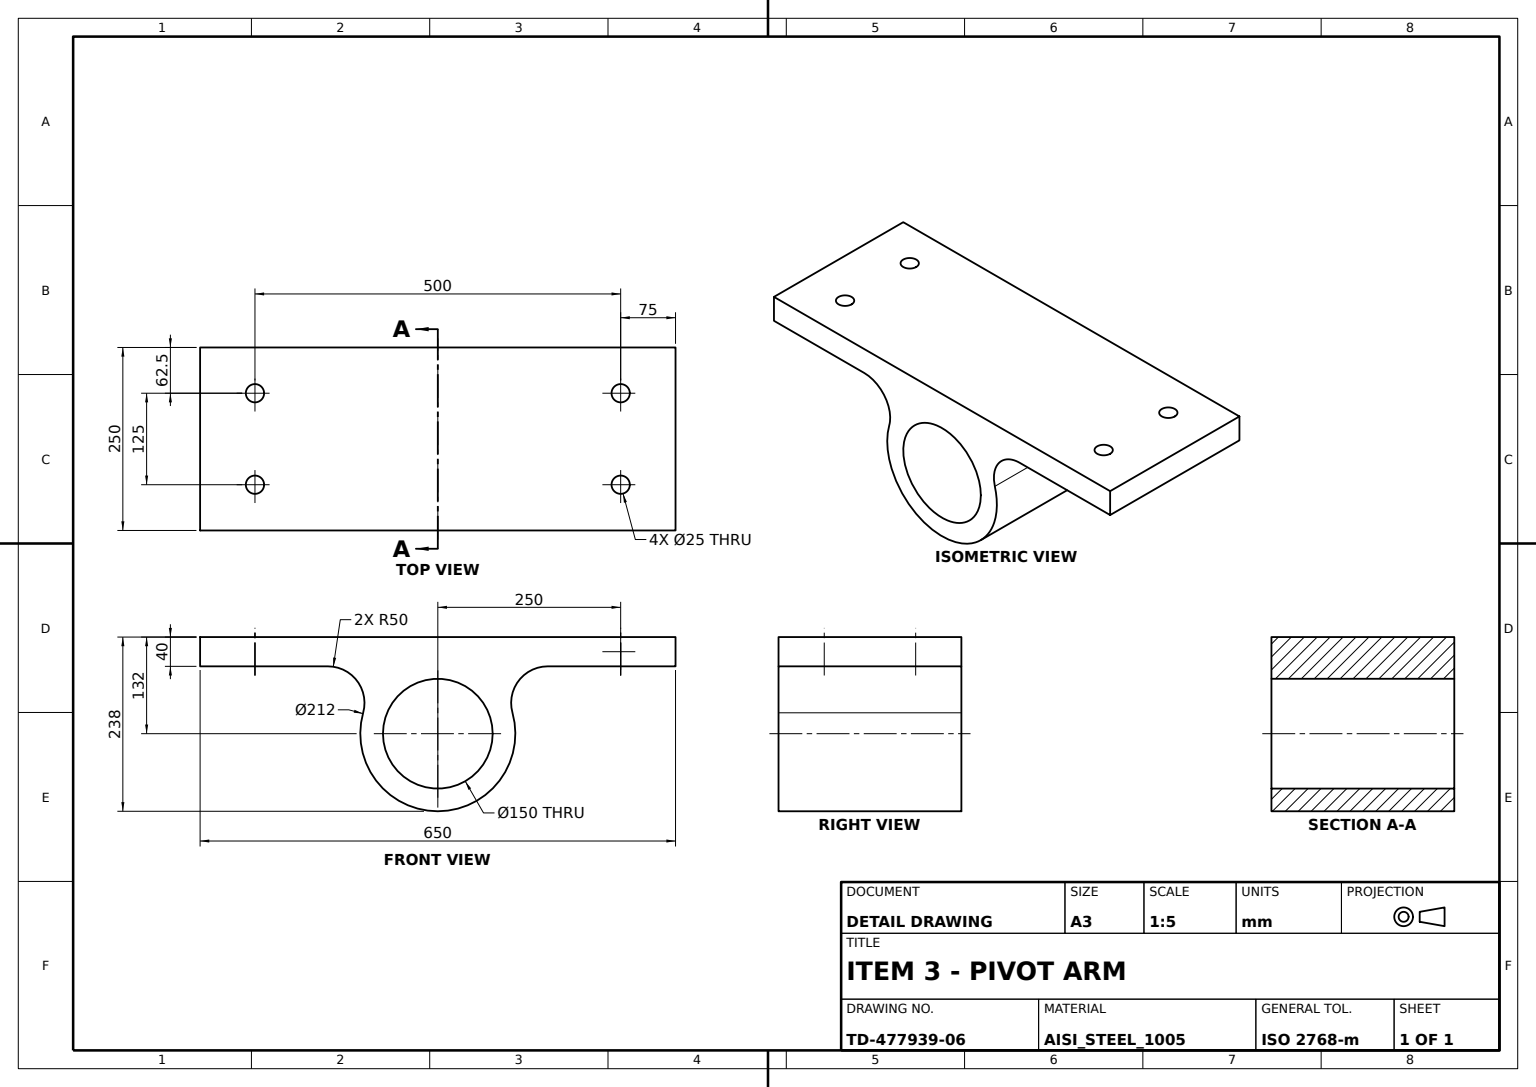
ISO-10303-21;
HEADER;
FILE_DESCRIPTION((''),'2;1');
FILE_NAME('','',(''),(''),'','','');
FILE_SCHEMA(('AUTOMOTIVE_DESIGN'));
ENDSEC;
DATA;
#1=APPLICATION_CONTEXT('');
#2=PRODUCT_CONTEXT('',#1,'mechanical');
#3=PRODUCT('','','',(#2));
#4=PRODUCT_DEFINITION_FORMATION('','',#3);
#5=PRODUCT_DEFINITION_CONTEXT('',#1,'design');
#6=PRODUCT_DEFINITION('','',#4,#5);
#7=PRODUCT_DEFINITION_SHAPE('','',#6);
#8=(LENGTH_UNIT()NAMED_UNIT(*)SI_UNIT(.MILLI.,.METRE.));
#9=(NAMED_UNIT(*)PLANE_ANGLE_UNIT()SI_UNIT($,.RADIAN.));
#10=(NAMED_UNIT(*)SI_UNIT($,.STERADIAN.)SOLID_ANGLE_UNIT());
#11=UNCERTAINTY_MEASURE_WITH_UNIT(LENGTH_MEASURE(0.005),#8,'distance_accuracy_value','');
#12=(GEOMETRIC_REPRESENTATION_CONTEXT(3)GLOBAL_UNCERTAINTY_ASSIGNED_CONTEXT((#11))GLOBAL_UNIT_ASSIGNED_CONTEXT((#8,#9,#10))REPRESENTATION_CONTEXT('',''));
#13=CARTESIAN_POINT('',(125.,-102.086024,28.538462));
#14=VERTEX_POINT('',#13);
#15=CARTESIAN_POINT('',(125.,102.086024,28.538462));
#16=VERTEX_POINT('',#15);
#17=CARTESIAN_POINT('',(125.,0.,0.));
#18=DIRECTION('',(1.,0.,0.));
#19=DIRECTION('',(0.,1.,0.));
#20=AXIS2_PLACEMENT_3D('',#17,#18,#19);
#21=CIRCLE('',#20,106.);
#22=EDGE_CURVE('',#14,#16,#21,.T.);
#23=ORIENTED_EDGE('',*,*,#22,.F.);
#24=CARTESIAN_POINT('',(-125.,-102.086024,28.538462));
#25=VERTEX_POINT('',#24);
#26=DIRECTION('',(-1.,0.,0.));
#27=VECTOR('',#26,1000.);
#28=LINE('',#13,#27);
#29=EDGE_CURVE('',#14,#25,#28,.T.);
#30=ORIENTED_EDGE('',*,*,#29,.T.);
#31=CARTESIAN_POINT('',(-125.,102.086024,28.538462));
#32=VERTEX_POINT('',#31);
#33=CARTESIAN_POINT('',(-125.,0.,0.));
#34=AXIS2_PLACEMENT_3D('',#33,#18,#19);
#35=CIRCLE('',#34,106.);
#36=EDGE_CURVE('',#25,#32,#35,.T.);
#37=ORIENTED_EDGE('',*,*,#36,.T.);
#38=LINE('',#15,#27);
#39=EDGE_CURVE('',#16,#32,#38,.T.);
#40=ORIENTED_EDGE('',*,*,#39,.F.);
#41=EDGE_LOOP('',(#23,#30,#37,#40));
#42=FACE_BOUND('',#41,.T.);
#43=DIRECTION('',(0.,0.,1.));
#44=AXIS2_PLACEMENT_3D('',#17,#26,#43);
#45=CYLINDRICAL_SURFACE('',#44,106.);
#46=ADVANCED_FACE('',(#42),#45,.T.);
#47=CARTESIAN_POINT('',(-125.,325.,132.));
#48=VERTEX_POINT('',#47);
#49=CARTESIAN_POINT('',(-125.,-325.,132.));
#50=VERTEX_POINT('',#49);
#51=DIRECTION('',(0.,-1.,0.));
#52=VECTOR('',#51,1000.);
#53=LINE('',#47,#52);
#54=EDGE_CURVE('',#48,#50,#53,.T.);
#55=ORIENTED_EDGE('',*,*,#54,.T.);
#56=CARTESIAN_POINT('',(125.,-325.,132.));
#57=VERTEX_POINT('',#56);
#58=LINE('',#56,#27);
#59=EDGE_CURVE('',#57,#50,#58,.T.);
#60=ORIENTED_EDGE('',*,*,#59,.F.);
#61=CARTESIAN_POINT('',(125.,325.,132.));
#62=VERTEX_POINT('',#61);
#63=LINE('',#61,#52);
#64=EDGE_CURVE('',#62,#57,#63,.T.);
#65=ORIENTED_EDGE('',*,*,#64,.F.);
#66=LINE('',#61,#27);
#67=EDGE_CURVE('',#62,#48,#66,.T.);
#68=ORIENTED_EDGE('',*,*,#67,.T.);
#69=EDGE_LOOP('',(#55,#60,#65,#68));
#70=FACE_BOUND('',#69,.T.);
#71=CARTESIAN_POINT('',(-62.5,-237.5,132.));
#72=VERTEX_POINT('',#71);
#73=CARTESIAN_POINT('',(-62.5,-250.,132.));
#74=AXIS2_PLACEMENT_3D('',#73,#43,#19);
#75=CIRCLE('',#74,12.5);
#76=EDGE_CURVE('',#72,#72,#75,.T.);
#77=ORIENTED_EDGE('',*,*,#76,.F.);
#78=EDGE_LOOP('',(#77));
#79=FACE_BOUND('',#78,.T.);
#80=CARTESIAN_POINT('',(62.5,-237.5,132.));
#81=VERTEX_POINT('',#80);
#82=CARTESIAN_POINT('',(62.5,-250.,132.));
#83=AXIS2_PLACEMENT_3D('',#82,#43,#19);
#84=CIRCLE('',#83,12.5);
#85=EDGE_CURVE('',#81,#81,#84,.T.);
#86=ORIENTED_EDGE('',*,*,#85,.F.);
#87=EDGE_LOOP('',(#86));
#88=FACE_BOUND('',#87,.T.);
#89=CARTESIAN_POINT('',(-62.5,262.5,132.));
#90=VERTEX_POINT('',#89);
#91=CARTESIAN_POINT('',(-62.5,250.,132.));
#92=AXIS2_PLACEMENT_3D('',#91,#43,#19);
#93=CIRCLE('',#92,12.5);
#94=EDGE_CURVE('',#90,#90,#93,.T.);
#95=ORIENTED_EDGE('',*,*,#94,.F.);
#96=EDGE_LOOP('',(#95));
#97=FACE_BOUND('',#96,.T.);
#98=CARTESIAN_POINT('',(62.5,262.5,132.));
#99=VERTEX_POINT('',#98);
#100=CARTESIAN_POINT('',(62.5,250.,132.));
#101=AXIS2_PLACEMENT_3D('',#100,#43,#19);
#102=CIRCLE('',#101,12.5);
#103=EDGE_CURVE('',#99,#99,#102,.T.);
#104=ORIENTED_EDGE('',*,*,#103,.F.);
#105=EDGE_LOOP('',(#104));
#106=FACE_BOUND('',#105,.T.);
#107=DIRECTION('',(0.,0.,-1.));
#108=AXIS2_PLACEMENT_3D('',#61,#107,#26);
#109=PLANE('',#108);
#110=ADVANCED_FACE('',(#70,#79,#88,#97,#106),#109,.F.);
#111=ORIENTED_EDGE('',*,*,#103,.T.);
#112=EDGE_LOOP('',(#111));
#113=FACE_BOUND('',#112,.T.);
#114=CARTESIAN_POINT('',(75.,250.,92.));
#115=VERTEX_POINT('',#114);
#116=CARTESIAN_POINT('',(62.5,250.,92.));
#117=AXIS2_PLACEMENT_3D('',#116,#43,#18);
#118=CIRCLE('',#117,12.5);
#119=EDGE_CURVE('',#115,#115,#118,.T.);
#120=ORIENTED_EDGE('',*,*,#119,.F.);
#121=EDGE_LOOP('',(#120));
#122=FACE_BOUND('',#121,.T.);
#123=CARTESIAN_POINT('',(62.5,250.,7.));
#124=AXIS2_PLACEMENT_3D('',#123,#43,#18);
#125=CYLINDRICAL_SURFACE('',#124,12.5);
#126=ADVANCED_FACE('',(#113,#122),#125,.F.);
#127=ORIENTED_EDGE('',*,*,#119,.T.);
#128=EDGE_LOOP('',(#127));
#129=FACE_BOUND('',#128,.T.);
#130=CARTESIAN_POINT('',(-50.,250.,92.));
#131=VERTEX_POINT('',#130);
#132=CARTESIAN_POINT('',(-62.5,250.,92.));
#133=AXIS2_PLACEMENT_3D('',#132,#43,#18);
#134=CIRCLE('',#133,12.5);
#135=EDGE_CURVE('',#131,#131,#134,.T.);
#136=ORIENTED_EDGE('',*,*,#135,.T.);
#137=EDGE_LOOP('',(#136));
#138=FACE_BOUND('',#137,.T.);
#139=CARTESIAN_POINT('',(125.,325.,92.));
#140=VERTEX_POINT('',#139);
#141=CARTESIAN_POINT('',(-125.,325.,92.));
#142=VERTEX_POINT('',#141);
#143=LINE('',#139,#27);
#144=EDGE_CURVE('',#140,#142,#143,.T.);
#145=ORIENTED_EDGE('',*,*,#144,.F.);
#146=CARTESIAN_POINT('',(125.,150.239808,92.));
#147=VERTEX_POINT('',#146);
#148=VECTOR('',#19,1000.);
#149=LINE('',#146,#148);
#150=EDGE_CURVE('',#147,#140,#149,.T.);
#151=ORIENTED_EDGE('',*,*,#150,.F.);
#152=CARTESIAN_POINT('',(-125.,150.239808,92.));
#153=VERTEX_POINT('',#152);
#154=LINE('',#146,#27);
#155=EDGE_CURVE('',#147,#153,#154,.T.);
#156=ORIENTED_EDGE('',*,*,#155,.T.);
#157=LINE('',#152,#148);
#158=EDGE_CURVE('',#153,#142,#157,.T.);
#159=ORIENTED_EDGE('',*,*,#158,.T.);
#160=EDGE_LOOP('',(#145,#151,#156,#159));
#161=FACE_BOUND('',#160,.T.);
#162=AXIS2_PLACEMENT_3D('',#146,#43,#18);
#163=PLANE('',#162);
#164=ADVANCED_FACE('',(#129,#138,#161),#163,.F.);
#165=ORIENTED_EDGE('',*,*,#59,.T.);
#166=CARTESIAN_POINT('',(-125.,-325.,92.));
#167=VERTEX_POINT('',#166);
#168=VECTOR('',#107,1000.);
#169=LINE('',#49,#168);
#170=EDGE_CURVE('',#50,#167,#169,.T.);
#171=ORIENTED_EDGE('',*,*,#170,.T.);
#172=CARTESIAN_POINT('',(125.,-325.,92.));
#173=VERTEX_POINT('',#172);
#174=LINE('',#172,#27);
#175=EDGE_CURVE('',#173,#167,#174,.T.);
#176=ORIENTED_EDGE('',*,*,#175,.F.);
#177=LINE('',#56,#168);
#178=EDGE_CURVE('',#57,#173,#177,.T.);
#179=ORIENTED_EDGE('',*,*,#178,.F.);
#180=EDGE_LOOP('',(#165,#171,#176,#179));
#181=FACE_BOUND('',#180,.T.);
#182=AXIS2_PLACEMENT_3D('',#56,#19,#43);
#183=PLANE('',#182);
#184=ADVANCED_FACE('',(#181),#183,.F.);
#185=VECTOR('',#43,1000.);
#186=LINE('',#141,#185);
#187=EDGE_CURVE('',#142,#48,#186,.T.);
#188=ORIENTED_EDGE('',*,*,#187,.T.);
#189=ORIENTED_EDGE('',*,*,#67,.F.);
#190=LINE('',#139,#185);
#191=EDGE_CURVE('',#140,#62,#190,.T.);
#192=ORIENTED_EDGE('',*,*,#191,.F.);
#193=ORIENTED_EDGE('',*,*,#144,.T.);
#194=EDGE_LOOP('',(#188,#189,#192,#193));
#195=FACE_BOUND('',#194,.T.);
#196=AXIS2_PLACEMENT_3D('',#139,#51,#107);
#197=PLANE('',#196);
#198=ADVANCED_FACE('',(#195),#197,.F.);
#199=ORIENTED_EDGE('',*,*,#85,.T.);
#200=EDGE_LOOP('',(#199));
#201=FACE_BOUND('',#200,.T.);
#202=CARTESIAN_POINT('',(75.,-250.,92.));
#203=VERTEX_POINT('',#202);
#204=CARTESIAN_POINT('',(62.5,-250.,92.));
#205=AXIS2_PLACEMENT_3D('',#204,#43,#18);
#206=CIRCLE('',#205,12.5);
#207=EDGE_CURVE('',#203,#203,#206,.T.);
#208=ORIENTED_EDGE('',*,*,#207,.F.);
#209=EDGE_LOOP('',(#208));
#210=FACE_BOUND('',#209,.T.);
#211=CARTESIAN_POINT('',(62.5,-250.,7.));
#212=AXIS2_PLACEMENT_3D('',#211,#43,#18);
#213=CYLINDRICAL_SURFACE('',#212,12.5);
#214=ADVANCED_FACE('',(#201,#210),#213,.F.);
#215=CARTESIAN_POINT('',(125.,75.,0.));
#216=VERTEX_POINT('',#215);
#217=AXIS2_PLACEMENT_3D('',#17,#26,#19);
#218=CIRCLE('',#217,75.);
#219=EDGE_CURVE('',#216,#216,#218,.T.);
#220=ORIENTED_EDGE('',*,*,#219,.F.);
#221=EDGE_LOOP('',(#220));
#222=FACE_BOUND('',#221,.T.);
#223=CARTESIAN_POINT('',(-125.,75.,0.));
#224=VERTEX_POINT('',#223);
#225=AXIS2_PLACEMENT_3D('',#33,#26,#19);
#226=CIRCLE('',#225,75.);
#227=EDGE_CURVE('',#224,#224,#226,.T.);
#228=ORIENTED_EDGE('',*,*,#227,.T.);
#229=EDGE_LOOP('',(#228));
#230=FACE_BOUND('',#229,.T.);
#231=CYLINDRICAL_SURFACE('',#44,75.);
#232=ADVANCED_FACE('',(#222,#230),#231,.F.);
#233=ORIENTED_EDGE('',*,*,#135,.F.);
#234=EDGE_LOOP('',(#233));
#235=FACE_BOUND('',#234,.T.);
#236=ORIENTED_EDGE('',*,*,#94,.T.);
#237=EDGE_LOOP('',(#236));
#238=FACE_BOUND('',#237,.T.);
#239=CARTESIAN_POINT('',(-62.5,250.,7.));
#240=AXIS2_PLACEMENT_3D('',#239,#43,#18);
#241=CYLINDRICAL_SURFACE('',#240,12.5);
#242=ADVANCED_FACE('',(#235,#238),#241,.F.);
#243=ORIENTED_EDGE('',*,*,#207,.T.);
#244=EDGE_LOOP('',(#243));
#245=FACE_BOUND('',#244,.T.);
#246=CARTESIAN_POINT('',(-50.,-250.,92.));
#247=VERTEX_POINT('',#246);
#248=CARTESIAN_POINT('',(-62.5,-250.,92.));
#249=AXIS2_PLACEMENT_3D('',#248,#43,#18);
#250=CIRCLE('',#249,12.5);
#251=EDGE_CURVE('',#247,#247,#250,.T.);
#252=ORIENTED_EDGE('',*,*,#251,.T.);
#253=EDGE_LOOP('',(#252));
#254=FACE_BOUND('',#253,.T.);
#255=ORIENTED_EDGE('',*,*,#175,.T.);
#256=CARTESIAN_POINT('',(-125.,-150.239808,92.));
#257=VERTEX_POINT('',#256);
#258=LINE('',#166,#148);
#259=EDGE_CURVE('',#167,#257,#258,.T.);
#260=ORIENTED_EDGE('',*,*,#259,.T.);
#261=CARTESIAN_POINT('',(125.,-150.239808,92.));
#262=VERTEX_POINT('',#261);
#263=LINE('',#261,#27);
#264=EDGE_CURVE('',#262,#257,#263,.T.);
#265=ORIENTED_EDGE('',*,*,#264,.F.);
#266=LINE('',#172,#148);
#267=EDGE_CURVE('',#173,#262,#266,.T.);
#268=ORIENTED_EDGE('',*,*,#267,.F.);
#269=EDGE_LOOP('',(#255,#260,#265,#268));
#270=FACE_BOUND('',#269,.T.);
#271=AXIS2_PLACEMENT_3D('',#172,#43,#18);
#272=PLANE('',#271);
#273=ADVANCED_FACE('',(#245,#254,#270),#272,.F.);
#274=ORIENTED_EDGE('',*,*,#251,.F.);
#275=EDGE_LOOP('',(#274));
#276=FACE_BOUND('',#275,.T.);
#277=ORIENTED_EDGE('',*,*,#76,.T.);
#278=EDGE_LOOP('',(#277));
#279=FACE_BOUND('',#278,.T.);
#280=CARTESIAN_POINT('',(-62.5,-250.,7.));
#281=AXIS2_PLACEMENT_3D('',#280,#43,#18);
#282=CYLINDRICAL_SURFACE('',#281,12.5);
#283=ADVANCED_FACE('',(#276,#279),#282,.F.);
#284=ORIENTED_EDGE('',*,*,#219,.T.);
#285=EDGE_LOOP('',(#284));
#286=FACE_BOUND('',#285,.T.);
#287=ORIENTED_EDGE('',*,*,#191,.T.);
#288=ORIENTED_EDGE('',*,*,#64,.T.);
#289=ORIENTED_EDGE('',*,*,#178,.T.);
#290=ORIENTED_EDGE('',*,*,#267,.T.);
#291=CARTESIAN_POINT('',(125.,-150.239808,42.));
#292=AXIS2_PLACEMENT_3D('',#291,#26,#19);
#293=CIRCLE('',#292,50.);
#294=EDGE_CURVE('',#262,#14,#293,.T.);
#295=ORIENTED_EDGE('',*,*,#294,.T.);
#296=ORIENTED_EDGE('',*,*,#22,.T.);
#297=CARTESIAN_POINT('',(125.,150.239808,42.));
#298=AXIS2_PLACEMENT_3D('',#297,#26,#19);
#299=CIRCLE('',#298,50.);
#300=EDGE_CURVE('',#16,#147,#299,.T.);
#301=ORIENTED_EDGE('',*,*,#300,.T.);
#302=ORIENTED_EDGE('',*,*,#150,.T.);
#303=EDGE_LOOP('',(#287,#288,#289,#290,#295,#296,#301,#302));
#304=FACE_BOUND('',#303,.T.);
#305=AXIS2_PLACEMENT_3D('',#291,#26,#43);
#306=PLANE('',#305);
#307=ADVANCED_FACE('',(#286,#304),#306,.F.);
#308=ORIENTED_EDGE('',*,*,#29,.F.);
#309=ORIENTED_EDGE('',*,*,#294,.F.);
#310=ORIENTED_EDGE('',*,*,#264,.T.);
#311=CARTESIAN_POINT('',(-125.,-150.239808,42.));
#312=AXIS2_PLACEMENT_3D('',#311,#26,#19);
#313=CIRCLE('',#312,50.);
#314=EDGE_CURVE('',#257,#25,#313,.T.);
#315=ORIENTED_EDGE('',*,*,#314,.T.);
#316=EDGE_LOOP('',(#308,#309,#310,#315));
#317=FACE_BOUND('',#316,.T.);
#318=CYLINDRICAL_SURFACE('',#305,50.);
#319=ADVANCED_FACE('',(#317),#318,.F.);
#320=ORIENTED_EDGE('',*,*,#300,.F.);
#321=ORIENTED_EDGE('',*,*,#39,.T.);
#322=CARTESIAN_POINT('',(-125.,150.239808,42.));
#323=AXIS2_PLACEMENT_3D('',#322,#26,#19);
#324=CIRCLE('',#323,50.);
#325=EDGE_CURVE('',#32,#153,#324,.T.);
#326=ORIENTED_EDGE('',*,*,#325,.T.);
#327=ORIENTED_EDGE('',*,*,#155,.F.);
#328=EDGE_LOOP('',(#320,#321,#326,#327));
#329=FACE_BOUND('',#328,.T.);
#330=AXIS2_PLACEMENT_3D('',#297,#26,#43);
#331=CYLINDRICAL_SURFACE('',#330,50.);
#332=ADVANCED_FACE('',(#329),#331,.F.);
#333=ORIENTED_EDGE('',*,*,#227,.F.);
#334=EDGE_LOOP('',(#333));
#335=FACE_BOUND('',#334,.T.);
#336=ORIENTED_EDGE('',*,*,#314,.F.);
#337=ORIENTED_EDGE('',*,*,#259,.F.);
#338=ORIENTED_EDGE('',*,*,#170,.F.);
#339=ORIENTED_EDGE('',*,*,#54,.F.);
#340=ORIENTED_EDGE('',*,*,#187,.F.);
#341=ORIENTED_EDGE('',*,*,#158,.F.);
#342=ORIENTED_EDGE('',*,*,#325,.F.);
#343=ORIENTED_EDGE('',*,*,#36,.F.);
#344=EDGE_LOOP('',(#336,#337,#338,#339,#340,#341,#342,#343));
#345=FACE_BOUND('',#344,.T.);
#346=AXIS2_PLACEMENT_3D('',#311,#26,#43);
#347=PLANE('',#346);
#348=ADVANCED_FACE('',(#335,#345),#347,.T.);
#349=CLOSED_SHELL('',(#46,#110,#126,#164,#184,#198,#214,#232,#242,#273,#283,#307,#319,#332,#348));
#350=MANIFOLD_SOLID_BREP('',#349);
#351=ADVANCED_BREP_SHAPE_REPRESENTATION('',(#350),#12);
#352=SHAPE_DEFINITION_REPRESENTATION(#7,#351);
ENDSEC;
END-ISO-10303-21;
